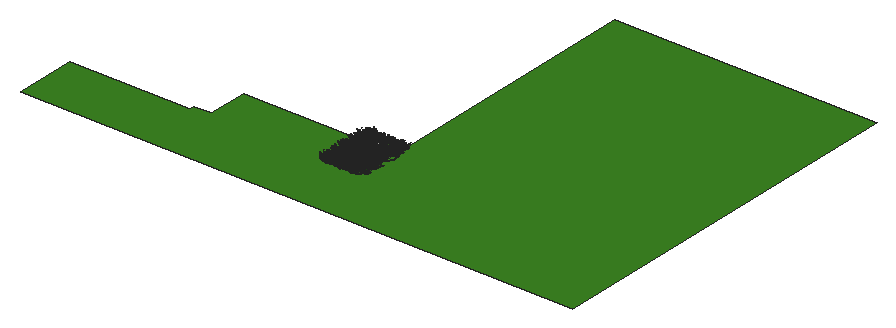
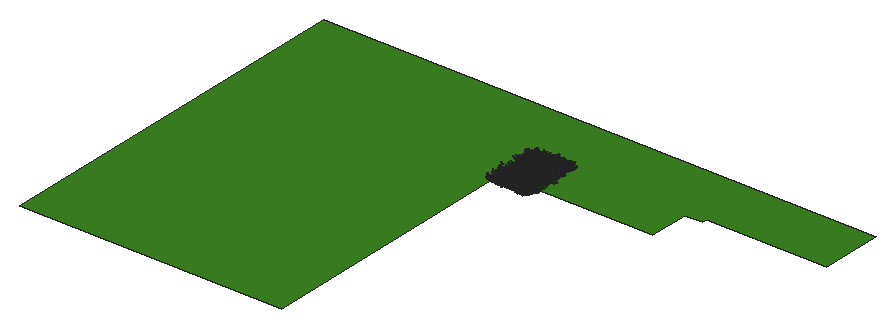
# SketchUp Ruby script. Lengths in inches.
U = 1.inch
M = Sketchup.active_model
def pt(a) = Geom::Point3d.new(a.map { |v| v * U })
def face(e, loops, mat)
  f = e.add_face(loops[0].map { |a| pt(a) })
  loops[1..].each { |l| e.add_face(l.map { |a| pt(a) }).erase! }
  f.material = f.back_material = mat if mat
  f
end
# faces: each face lists its corners as indices into pts; further lists are holes
def faces(e, pts, list, mat = nil) = list.each { |f| face(e, (f[0].is_a?(Array) ? f : [f]).map { |l| l.map { |i| pts[i] } }, mat) }
# xy, xz, yz: faces in a plane at the given z, y or x. An outline is a flat list of corners, or four numbers for a rectangle; further outlines are holes
def ring(l) = l.size == 4 ? [[l[0], l[1]], [l[2], l[1]], [l[2], l[3]], [l[0], l[3]]] : l.each_slice(2).to_a
def flat(e, list, mat, &to3) = list.each { |f| face(e, (f[0].is_a?(Array) ? f : [f]).map { |l| ring(l).map { |u, v| to3.(u, v) } }, mat) }
def xy(e, z, list, mat = nil) = flat(e, list, mat) { |x, y| [x, y, z] }
def xz(e, y, list, mat = nil) = flat(e, list, mat) { |x, z| [x, y, z] }
def yz(e, x, list, mat = nil) = flat(e, list, mat) { |y, z| [x, y, z] }
def lines(e, pts, list) = list.each { |a, b| e.add_line(pt(pts[a]), pt(pts[b])) }
# prism: a flat outline (further loops are holes) pulled along v
def prism(e, loops, v, mat = nil)
  f = face(e, loops, mat); d = Geom::Vector3d.new(v.map { |x| x * U })
  f.pushpull(f.normal.samedirection?(d) ? d.length : -d.length)
end
def box(e, o, s, mat = nil) = prism(e, [[o, [o[0] + s[0], o[1], o[2]], [o[0] + s[0], o[1] + s[1], o[2]], [o[0], o[1] + s[1], o[2]]]], [0, 0, s[2]], mat)
def at(x, y, z, deg = 0) = Geom::Transformation.translation(pt([x, y, z])) * Geom::Transformation.rotation(ORIGIN, Z_AXIS, deg.degrees)
def axes(o, x, y, z) = Geom::Transformation.new([*x, 0, *y, 0, *z, 0, *pt(o).to_a, 1])
def part(name) = M.definitions.add(name)
# library, detail: a bought-in or finely detailed component or shape, given as its bounding box
def library(name, o, s) = part(name).tap { |d| box(d.entities, o, s) }
def detail(e, o, s) = box(e.add_group.entities, o, s)
def put(e, d, t, mat = nil) = e.add_instance(d, t).tap { |i| i.material = mat if mat }
def group(e, t, mat = nil) = e.add_group.tap { |g| g.transformation = t; g.material = mat if mat }.entities
root = M.entities
M.materials.add("Material82").color = [68, 110, 58]
M.materials.add("Material83").color = [48, 90, 38]
M.materials.add("Material84").color = [68, 110, 48]
M.materials.add("Material85").color = [48, 90, 48]
M.materials.add("Material86").color = [58, 110, 58]
M.materials.add("Material87").color = [58, 90, 38]
M.materials.add("Material88").color = [68, 100, 58]
M.materials.add("Material89").color = [48, 100, 38]
M.materials.add("[Color M01]").color = [60, 133, 34]
c1 = part("grass00")
p = [[-0.6875,0.15,0],[-0.56,0.08,5.52],[-0.04,0.03,2.76],[0.48,-0.02,0],[0.35,-0.02,5.52],[-0.1,-0.14,5.52],
  [-0.12,0.65,8.37],[-0.42,0.65,8.37]]
faces(c1.entities,p,[[0,1,2,3],[3,2,4],[1,5,2],[5,4,2],[1,6,5],[4,5,6],[7,6,1]])
c2 = part("Group16\#1")
put(c2.entities,c1,axes([1.44,-0.61,-0.01],[0.05352,0.12609,0],[-0.10704,0.04543,0.07239],[0.06664,-0.02828,0.11628]),"Material85")
put(c2.entities,c1,axes([0.76,-0.15,-0.01],[0.04676,0.24062,0],[-0.23162,0.04501,0.06642],[0.0652,-0.01267,0.23595]),"Material82")
put(c2.entities,c1,axes([0.79,0.01,-0.01],[-0.00606,0.34651,0],[-0.34381,-0.00602,0.0432],[0.04319,0.00076,0.34386]))
put(c2.entities,c1,axes([1,0.23,-0.01],[-0.07192,0.31144,0],[-0.28722,-0.06632,0.1236],[0.12043,0.02781,0.29478]),"Material84")
put(c2.entities,c1,axes([1.66,0.77,-0.01],[-0.13828,0.29651,0],[-0.21551,-0.1005,0.22471],[0.20365,0.09498,0.23779]),"Material89")
put(c2.entities,c1,axes([0.6875,0.52,-0.01],[-0.18126,0.24051,0],[-0.22746,-0.17142,0.09788],[0.07817,0.05891,0.28481]),"Material84")
put(c2.entities,c1,axes([0.68,0.78,-0.01],[-0.215,0.18688,0],[-0.12385,-0.14248,0.21334],[0.13995,0.16101,0.18878]),"Material82")
put(c2.entities,c1,axes([0.56,1,-0.01],[-0.13756,0.07624,0],[-0.06159,-0.11112,0.0927],[0.04494,0.08108,0.12705]),"Material84")
put(c2.entities,c1,axes([0.2,0.64,-0.01],[-0.23729,0.07254,0],[-0.05711,-0.18681,0.153],[0.04473,0.14632,0.19535]),"Material89")
put(c2.entities,c1,axes([0.0625,0.72,-0.01],[-0.28874,0.02525,0],[-0.02179,-0.24916,0.14647],[0.01276,0.14591,0.25012]),"Material82")
put(c2.entities,c1,axes([-0.08,0.62,-0.01],[-0.34089,-0.04187,0],[0.03255,-0.26504,0.216],[-0.02633,0.21439,0.26703]),"Material89")
put(c2.entities,c1,axes([-0.34,0.98,-0.01],[-0.14314,-0.0493,0],[0.04397,-0.12769,0.06843],[-0.02228,0.0647,0.13505]),"Material89")
put(c2.entities,c1,axes([-0.87,1.45,-0.01],[-0.23488,-0.14114,0],[0.13761,-0.22901,0.06087],[-0.03135,0.05217,0.26717]))
put(c2.entities,c1,axes([-0.72,0.77,-0.01],[-0.14208,-0.13251,0],[0.07209,-0.0773,0.16301],[-0.11118,0.11922,0.1057]),"Material89")
put(c2.entities,c1,axes([-0.62,0.43,-0.01],[-0.14845,-0.21203,0],[0.18654,-0.13061,0.12304],[-0.10079,0.07057,0.22772]),"Material82")
put(c2.entities,c1,axes([-0.68,0.29,-0.01],[-0.13639,-0.32136,0],[0.31723,-0.13464,0.05579],[-0.05136,0.0218,0.34462]),"Material83")
put(c2.entities,c1,axes([-0.64,0.125,-0.01],[-0.0458,-0.23569,0],[0.22124,-0.043,0.08276],[-0.08124,0.01579,0.22538]),"Material86")
put(c2.entities,c1,axes([-1.6,-0.03,-0.01],[0.00576,-0.32897,0],[0.27526,0.00482,0.18018],[-0.18015,-0.00315,0.2753]),"Material84")
put(c2.entities,c1,axes([-1.36,-0.31,-0.01],[0.05718,-0.24765,0],[0.18172,0.04196,0.17267],[-0.16825,-0.03885,0.1865]),"Material89")
put(c2.entities,c1,axes([-1.54,-0.72,-0.01],[0.06537,-0.14017,0],[0.13555,0.06321,0.03939],[-0.0357,-0.01665,0.14956]))
put(c2.entities,c1,axes([-1.19,-0.9,-0.01],[0.09597,-0.12735,0],[0.11214,0.08451,0.07557],[-0.06035,-0.04548,0.14042]),"Material88")
put(c2.entities,c1,axes([-0.47,-0.54,-0.01],[0.11588,-0.10072,0],[0.0618,0.0711,0.12124],[-0.07953,-0.0915,0.0942]))
put(c2.entities,c1,axes([-0.47,-0.84,-0.01],[0.11927,-0.0661,0],[0.06603,0.11913,0.00646],[-0.00313,-0.00565,0.13621]),"Material84")
put(c2.entities,c1,axes([-0.38,-1.24,-0.01],[0.28037,-0.08571,0],[0.0618,0.20215,0.20315],[-0.05939,-0.19428,0.21139]),"Material88")
put(c2.entities,c1,axes([-0.06,-0.66,-0.01],[0.22719,-0.01987,0],[0.01247,0.14255,0.17758],[-0.01547,-0.17691,0.1431]),"Material87")
put(c2.entities,c1,axes([0.11,-0.89,-0.01],[0.14882,0.01828,0],[-0.01058,0.08611,0.12229],[0.01491,-0.12138,0.08676]),"Material85")
put(c2.entities,c1,axes([0.25,-0.72,-0.01],[0.20481,0.07053,0],[-0.06206,0.18022,0.10291],[0.03351,-0.0973,0.1906]),"Material85")
put(c2.entities,c1,axes([0.85,-1.42,-0.01],[0.16481,0.09904,0],[-0.09472,0.15762,0.05616],[0.02893,-0.04814,0.18389]),"Material84")
put(c2.entities,c1,axes([1.01,-1.09,-0.01],[0.21858,0.20385,0],[-0.17495,0.1876,0.15339],[0.10462,-0.11218,0.25652]),"Material89")
put(c2.entities,c1,axes([1.01,-0.71,-0.01],[0.08733,0.12473,0],[-0.06445,0.04512,0.13037],[0.1068,-0.07477,0.07867]),"Material85")
c3 = part("Group15\#1")
put(c3.entities,c2,at(0,0,0))
c4 = part("3darcstudiotree_grass00\#1")
put(c4.entities,c3,at(0,0,0))
xy(root,-29.74,[[486.07,932.5,1048.3125,932.5,1048.3125,1318.18,782.4375,1318.18,782.4375,1040.81,626.34,1040.81,626.34,1000.12,608.75,1000.12,608.75,994.94,486.07,994.94]],"[Color M01]")
put(root,c4,axes([747.01,1042.55,-29.74],[0.6827,1.82438,0],[-3.27697,0.19072,-0.00575],[-0.03023,0.00176,1.31904]))
put(root,c4,axes([747.21,997.3,-29.74],[0.45996,1.33665,0],[-3.57607,0.19139,-0.02967],[-0.17102,0.00915,1.57371]))
put(root,c4,axes([749.13,1041.28,-29.74],[-3.10229,-1.16988,0],[2.93363,-1.20992,-0.00934],[0.03186,-0.01314,1.57129]))
put(root,c4,axes([747.14,1024.93,-29.74],[2.66376,1.48543,0],[-3.56736,0.99495,-0.03132],[-0.13982,0.039,1.7905]))
put(root,c4,axes([749.33,1044.75,-29.74],[-2.84959,-0.68183,0],[2.166,-1.40791,-0.04577],[0.14869,-0.09665,1.96036]))
put(root,c4,axes([749.8125,1042.05,-29.74],[-4.12072,-0.27119,0],[0.6549,-1.54771,-0.03361],[0.02858,-0.06755,1.54092]))
put(root,c4,axes([749.8,996.66,-29.74],[-2.73846,-0.74739,0],[2.06192,-1.17502,-0.03348],[0.13147,-0.07492,1.87437]))
put(root,c4,axes([750.14,1027.05,-29.74],[-1.65449,-1.67632,0],[3.5536,-0.54549,-0.00938],[0.04968,-0.00763,1.62403]))
put(root,c4,axes([750.26,1016.8125,-29.74],[-2.10435,-1.3155,0],[3.64518,-0.9069,-0.04882],[0.17684,-0.044,1.38366]))
put(root,c4,axes([750.13,1033.6,-29.74],[-3.62624,-0.35306,0],[1.02554,-1.63824,-0.03453],[0.0374,-0.05975,1.44935]))
put(root,c4,axes([749.03,1039.09,-29.74],[0.82539,1.5958,0],[-3.41483,0.2747,-0.03877],[-0.28197,0.02268,1.93915]))
put(root,c4,axes([749.41,1011.43,-29.74],[3.93831,-0.79818,0],[2.14355,1.64496,-0.04443],[0.08068,0.06192,1.39643]))
put(root,c4,axes([750.67,1020.12,-29.74],[-2.03778,-1.0951,0],[3.7049,-1.07224,-0.05528],[0.23064,-0.06675,1.78248]))
put(root,c4,axes([750.68,1019.15,-29.74],[-3.67688,-0.6634,0],[1.45076,-1.25058,-0.02741],[0.08145,-0.07021,1.86713]))
put(root,c4,axes([749.05,1023.27,-29.74],[3.8654,0.35733,0],[-0.81256,1.36706,-0.007],[-0.00937,0.01576,1.56436]))
put(root,c4,axes([749.31,1029.81,-29.74],[0.38941,1.44392,0],[-4.06327,0.17043,-0.05804],[-0.26328,0.01104,1.39706]))
put(root,c4,axes([749.3,1050.98,-29.74],[3.44355,0.26807,0],[-0.70938,1.41724,-0.02055],[-0.0272,0.05435,1.87683]))
put(root,c4,axes([751.07,1007.75,-29.74],[-3.021,-0.6477,0],[1.60996,-1.16789,-0.02167],[0.0547,-0.03968,1.33527]))
put(root,c4,axes([750.93,1036.58,-29.74],[-4.07234,0.0884,0],[-0.21728,-1.55677,-0.00024],[-0.00008,-0.0006,1.85086]))
put(root,c4,axes([750.67,999.31,-29.74],[-3.52536,0.66718,0],[-1.57507,-1.29441,-0.02803],[-0.08559,-0.07034,1.92571]))
put(root,c4,axes([749.79,1053.3125,-29.74],[0.25287,1.52902,0],[-3.62555,0.09325,-0.03468],[-0.21891,0.00563,1.72254]))
put(root,c4,axes([750.23,1014.4375,-29.74],[3.86172,-0.56351,0],[1.21864,1.29888,-0.04569],[0.10723,0.11428,1.78027]))
put(root,c4,axes([751.52,1049.22,-29.74],[-4.49885,0.1512,0],[-0.3136,-1.45126,-0.04489],[-0.02566,-0.11876,1.86365]))
put(root,c4,axes([751.02,1009.58,-29.74],[2.47969,-0.8558,0],[2.79846,1.26111,-0.0129],[0.03707,0.01671,1.39029]))
put(root,c4,axes([750.74,1025.95,-29.74],[3.77184,-0.74152,0],[2.04611,1.61872,-0.00236],[0.0043,0.00341,1.40454]))
put(root,c4,axes([751.9375,1047.68,-29.74],[-3.95195,-0.11479,0],[0.31612,-1.69258,-0.00991],[0.00383,-0.02049,1.69565]))
put(root,c4,axes([750.69,1003.09,-29.74],[4.4523,-0.10128,0],[0.21715,1.4846,-0.03809],[0.01394,0.09529,1.79573]))
put(root,c4,axes([751.125,1001.68,-29.74],[3.96943,-0.89247,0],[1.86138,1.2876,-0.05304],[0.17378,0.12021,1.86337]))
put(root,c4,axes([752.54,1005.29,-29.74],[-0.06079,-1.40056,0],[3.30003,-0.02228,-0.01279],[0.0855,-0.00058,1.65408]))
put(root,c4,axes([752.48,1031.88,-29.74],[-0.47592,1.56401,0],[-3.26389,-0.15447,-0.01529],[-0.10295,-0.00487,1.67142]))
put(root,c4,axes([754.48,1006.18,-29.74],[-0.30634,-1.35211,0],[4.22133,-0.14875,-0.01785],[0.10663,-0.00376,1.90542]))
put(root,c4,axes([754.57,1006.96,-29.74],[0.00917,-1.7323,0],[3.83355,0.00316,-0.00952],[0.04811,0.00004,1.45276]))
put(root,c4,axes([755.09,1031.06,-29.74],[-3.94041,-0.17555,0],[0.52244,-1.82386,-0.03054],[0.01805,-0.06303,1.83699]))
put(root,c4,axes([755.2,1038.49,-29.74],[-3.62534,0.37466,0],[-0.93047,-1.40031,-0.00505],[-0.0081,-0.01218,1.74136]))
put(root,c4,axes([754.51,1022.87,-29.74],[3.51422,-0.54071,0],[1.19989,1.21289,-0.03886],[0.08676,0.0877,1.52001]))
put(root,c4,axes([756.16,1051.37,-29.74],[-3.51186,-0.721,0],[1.80955,-1.37083,-0.02288],[0.05511,-0.04175,1.53217]))
put(root,c4,axes([756.18,1029.875,-29.74],[1.44921,-1.37247,0],[3.47001,0.56986,-0.04485],[0.23379,0.03839,1.59096]))
put(root,c4,axes([755.31,1002.98,-29.74],[0.66388,1.42145,0],[-3.998,0.29041,-0.0472],[-0.22325,0.01622,1.46547]))
put(root,c4,axes([755.41,1025.51,-29.74],[2.60904,1.49403,0],[-2.88542,0.78369,-0.04649],[-0.18984,0.05156,1.30192]))
put(root,c4,axes([755.52,1013.72,-29.74],[3.83063,0.28141,0],[-0.63066,1.33518,-0.03922],[-0.04064,0.08605,1.46066]))
put(root,c4,axes([756.07,1028.07,-29.74],[2.98326,-0.56932,0],[1.56375,1.27443,-0.0104],[0.02417,0.0197,1.43546]))
put(root,c4,axes([755.47,1039.72,-29.74],[0.44153,1.60869,0],[-4.59886,0.19631,-0.03135],[-0.13775,0.00588,1.53244]))
put(root,c4,axes([756.1,1042.45,-29.74],[3.7963,-0.32727,0],[0.82791,1.49367,-0.02018],[0.02229,0.04022,1.50307]))
put(root,c4,axes([758.06,1018.1,-29.74],[-2.44222,-1.21448,0],[3.27109,-1.02306,-0.01126],[0.03735,-0.01168,1.32461]))
put(root,c4,axes([757.73,1012.8,-29.74],[-3.39135,-0.3159,0],[0.83318,-1.39116,-0.01801],[0.02035,-0.03397,1.33554]))
put(root,c4,axes([757.61,1009.53,-29.74],[-1.25644,-1.35671,0],[3.16457,-0.45581,-0.03784],[0.23357,-0.03364,1.65933]))
put(root,c4,axes([758,1046.6,-29.74],[-0.2827,-1.72948,0],[4.63241,-0.11777,-0.03565],[0.15653,-0.00398,1.53082]))
put(root,c4,axes([758.16,1020.64,-29.74],[-4.6912,-0.24024,0],[0.57575,-1.74859,-0.02421],[0.01544,-0.0469,1.66024]))
put(root,c4,axes([757.25,1045.24,-29.74],[2.39093,-1.03283,0],[3.02488,1.08907,-0.05494],[0.24262,0.08735,1.83588]))
put(root,c4,axes([757.28,1001.06,-29.74],[3.97766,0.18345,0],[-0.40911,1.37962,-0.0104],[-0.00856,0.02886,1.87036]))
put(root,c4,axes([758.13,1036.82,-29.74],[2.63553,-1.14097,0],[3.49929,1.25715,-0.04921],[0.17097,0.06142,1.66765]))
put(root,c4,axes([758,1034.22,-29.74],[-2.26024,1.36544,0],[-3.77789,-0.97262,-0.02867],[-0.12669,-0.03262,1.78429]))
put(root,c4,axes([757.52,997.26,-29.74],[2.88281,0.64392,0],[-1.76321,1.22772,-0.02459],[-0.08623,0.06004,1.90817]))
put(root,c4,axes([758.22,1016.9375,-29.74],[3.80429,-0.95187,0],[2.21902,1.37934,-0.04672],[0.14892,0.09257,1.84728]))
put(root,c4,axes([757.61,998.35,-29.74],[3.38308,1.28097,0],[-3.13031,1.28579,-0.04664],[-0.1697,0.06971,1.77978]))
put(root,c4,axes([758.21,1048.77,-29.74],[1.17272,1.70605,0],[-3.75992,0.40197,-0.02312],[-0.1149,0.01228,1.50331]))
put(root,c4,axes([760.57,1020.29,-29.74],[2.08515,-1.11593,0],[3.14779,0.91479,-0.04551],[0.20545,0.05971,1.64335]))
put(root,c4,axes([760.6,1014.2,-29.74],[-2.84594,1.17329,0],[-3.06349,-1.15571,-0.01205],[-0.05136,-0.01938,1.87482]))
put(root,c4,axes([761.64,1004.18,-29.74],[-4.1718,-0.04402,0],[0.1133,-1.66995,-0.01377],[0.00192,-0.02825,1.65227]))
put(root,c4,axes([761.21,1028.09,-29.74],[-3.19418,0.83767,0],[-2.09756,-1.24397,-0.00165],[-0.00457,-0.00271,1.42237]))
put(root,c4,axes([762.15,1009.56,-29.74],[-3.23677,-0.61439,0],[2.0349,-1.66734,-0.00367],[0.00726,-0.00595,1.60507]))
put(root,c4,axes([761.77,1001.03,-29.74],[0.66157,-1.84804,0],[3.88634,0.21638,-0.01886],[0.11067,0.00616,1.74385]))
put(root,c4,axes([760.78,1024.71,-29.74],[3.70848,0.20038,0],[-0.48617,1.3994,-0.00884],[-0.00845,0.02433,1.89082]))
put(root,c4,axes([760.92,1049.92,-29.74],[3.47876,0.69717,0],[-2.07434,1.60981,-0.02666],[-0.05222,0.04053,1.48409]))
put(root,c4,axes([761.49,998.35,-29.74],[-1.68767,1.14523,0],[-4.10192,-0.94014,-0.02835],[-0.11929,-0.02734,1.73088]))
put(root,c4,axes([762.9375,1042.89,-29.74],[-4.10821,-0.63147,0],[1.40621,-1.42285,-0.03755],[0.0732,-0.07407,1.55797]))
put(root,c4,axes([761.49,1039.9,-29.74],[4.36048,0.20882,0],[-0.42656,1.38529,-0.01966],[-0.01597,0.05186,1.78732]))
put(root,c4,axes([761.93,1031.31,-29.74],[-1.75851,1.2095,0],[-3.69968,-0.83659,-0.01882],[-0.09945,-0.02249,1.94745]))
put(root,c4,axes([763.47,1038.96,-29.74],[-1.44336,-1.26835,0],[3.91991,-0.69378,-0.01184],[0.05292,-0.00937,1.57815]))
put(root,c4,axes([763.24,1044.71,-29.74],[-0.45128,-1.33361,0],[4.22591,-0.22241,-0.03174],[0.17504,-0.00921,1.77768]))
put(root,c4,axes([762.29,1007.53,-29.74],[3.82795,-0.89848,0],[2.12017,1.40489,-0.02674],[0.0662,0.04387,1.50406]))
put(root,c4,axes([763.36,1047.18,-29.74],[-2.48368,-1.57939,0],[3.38438,-0.82775,-0.05324],[0.27998,-0.06848,1.84703]))
put(root,c4,axes([763.24,1022.47,-29.74],[-3.70161,0.1835,0],[-0.55617,-1.74492,-0.04842],[-0.0352,-0.11043,1.94818]))
put(root,c4,axes([763.78,996.95,-29.74],[-2.02199,-1.57321,0],[3.0284,-0.60536,-0.03791],[0.25064,-0.0501,1.88609]))
put(root,c4,axes([762.4375,1019.16,-29.74],[4.60425,0.18746,0],[-0.4763,1.81947,-0.06196],[-0.02818,0.10763,1.53928]))
put(root,c4,axes([762.65,1005.1,-29.74],[3.66376,0.25232,0],[-0.75626,1.7079,-0.04039],[-0.02947,0.06656,1.39779]))
put(root,c4,axes([762.9,1016.97,-29.74],[3.38223,0.96892,0],[-2.45655,1.33368,-0.05492],[-0.16887,0.09168,1.63919]))
put(root,c4,axes([764.09,1050.81,-29.74],[-3.51929,1.02852,0],[-2.47816,-1.3188,-0.03727],[-0.13373,-0.07117,1.88005]))
put(root,c4,axes([763.54,1030.35,-29.74],[3.59827,-1.20315,0],[2.55541,1.18863,-0.04452],[0.1901,0.08842,1.95574]))
put(root,c4,axes([762.75,1034.56,-29.74],[2.55345,1.05656,0],[-3.3838,1.27189,-0.0237],[-0.06613,0.02486,1.35093]))
put(root,c4,axes([763.8,1012.71,-29.74],[3.17823,1.19717,0],[-2.46254,1.01678,-0.00574],[-0.02103,0.00868,1.41814]))
put(root,c4,axes([764,1036.57,-29.74],[1.4209,1.26091,0],[-3.92098,0.6872,-0.00487],[-0.02309,0.00405,1.66894]))
put(root,c4,axes([766.67,1001.15,-29.74],[-4.20115,-0.27572,0],[0.6063,-1.43684,-0.03971],[0.03476,-0.08238,1.4765]))
put(root,c4,axes([766.01,1047.37,-29.74],[-2.56197,0.85481,0],[-2.91428,-1.35846,-0.04396],[-0.15305,-0.07134,1.82298]))
put(root,c4,axes([766.08,1048.45,-29.74],[-3.07207,1.32257,0],[-2.98229,-1.07739,-0.02313],[-0.10886,-0.03933,1.93523]))
put(root,c4,axes([766.07,1007.88,-29.74],[3.03154,-1.30842,0],[2.70015,0.973,-0.04297],[0.17128,0.06172,1.48019]))
put(root,c4,axes([765.98,1010.51,-29.74],[4.0708,-0.43574,0],[1.12817,1.63922,-0.0215],[0.0298,0.0433,1.70776]))
put(root,c4,axes([765.75,1035.875,-29.74],[1.45585,1.40356,0],[-4.29762,0.69331,-0.06498],[-0.33385,0.05386,1.93183]))
put(root,c4,axes([766.31,1021.4,-29.74],[3.98961,-0.74286,0],[1.49364,1.24762,-0.01833],[0.03992,0.03334,1.33779]))
put(root,c4,axes([766.23,1023.45,-29.74],[-1.90909,1.29111,0],[-3.77719,-0.86865,-0.00159],[-0.00678,-0.00156,1.61385]))
put(root,c4,axes([766.16,1042.29,-29.74],[3.44974,0.13102,0],[-0.35474,1.45265,-0.03978],[-0.02715,0.11118,1.9745]))
put(root,c4,axes([766.79,1031.26,-29.74],[4.01141,-0.57098,0],[1.38004,1.50792,-0.00463],[0.00922,0.01007,1.7876]))
put(root,c4,axes([768.29,999.71,-29.74],[-2.56515,-0.8375,0],[2.7288,-1.2999,-0.02106],[0.06081,-0.02897,1.45262]))
put(root,c4,axes([766.27,1017.93,-29.74],[1.21271,1.28553,0],[-4.16441,0.61099,-0.01219],[-0.04469,0.00656,1.30286]))
put(root,c4,axes([767.52,1011.61,-29.74],[-3.04036,1.06501,0],[-2.34315,-1.04035,-0.02123],[-0.07304,-0.03243,1.37003]))
put(root,c4,axes([767.73,1017.28,-29.74],[1.27723,-1.67859,0],[3.60633,0.42678,-0.0465],[0.22987,0.0272,1.45674]))
put(root,c4,axes([766.8,1005.15,-29.74],[4.09443,-0.06366,0],[0.15428,1.54325,-0.03451],[0.00867,0.0867,1.8714]))
put(root,c4,axes([768.57,1051.75,-29.74],[-2.71598,-1.39793,0],[3.51357,-1.0617,-0.04805],[0.18587,-0.05616,1.61679]))
put(root,c4,axes([766.75,1003.16,-29.74],[3.43879,0.48398,0],[-1.47194,1.62658,-0.03925],[-0.05225,0.05774,1.29995]))
put(root,c4,axes([768.13,1044.11,-29.74],[0.94515,-1.66762,0],[4.07339,0.35906,-0.0396],[0.18346,0.01617,1.48525]))
put(root,c4,axes([767.67,1034.39,-29.74],[2.86215,-0.69885,0],[2.15737,1.37418,-0.03178],[0.09016,0.05743,1.65559]))
put(root,c4,axes([767.39,1039.95,-29.74],[2.07536,1.00802,0],[-2.97078,0.95128,-0.04172],[-0.20153,0.06453,1.78477]))
put(root,c4,axes([768.93,1037.93,-29.74],[0.03648,-1.32003,0],[3.51668,0.01511,-0.01263],[0.08154,0.00035,1.70174]))
put(root,c4,axes([769.15,1013.93,-29.74],[-0.06785,-1.57512,0],[4.70678,-0.03153,-0.0635],[0.34719,-0.00233,1.92948]))
put(root,c4,axes([768.79,1027.73,-29.74],[-0.80195,1.7338,0],[-4.65742,-0.33505,-0.02378],[-0.12913,-0.00929,1.95907]))
put(root,c4,axes([769.1,997.23,-29.74],[-1.48177,1.26839,0],[-3.97677,-0.72256,-0.00587],[-0.02393,-0.00435,1.47291]))
put(root,c4,axes([769.13,1028.88,-29.74],[4.46941,0.03034,0],[-0.07094,1.62545,-0.04862],[-0.00377,0.08633,1.39123]))
put(root,c4,axes([769.6,1024.98,-29.74],[3.5964,-0.66598,0],[1.43149,1.20228,-0.03796],[0.09777,0.08212,1.52986]))
put(root,c4,axes([771.54,1007.8,-29.74],[-3.83088,0.01586,0],[-0.04003,-1.50367,-0.01485],[-0.00089,-0.03334,1.62647]))
put(root,c4,axes([771.44,1036.53,-29.74],[2.50638,-0.90958,0],[2.96207,1.26944,-0.00074],[0.00258,0.00111,1.68668]))
put(root,c4,axes([772.05,1021.55,-29.74],[-1.26463,-1.25515,0],[3.81596,-0.59798,-0.04918],[0.19961,-0.03128,1.34418]))
put(root,c4,axes([771.48,1029.59,-29.74],[-2.59269,1.36416,0],[-3.43206,-1.0145,-0.01976],[-0.08545,-0.02526,1.7373]))
put(root,c4,axes([771.25,1031.63,-29.74],[4.23995,-0.14734,0],[0.39715,1.77755,-0.00682],[0.00263,0.01179,1.49182]))
put(root,c4,axes([772.49,1023.46,-29.74],[0.54946,-1.30633,0],[4.42126,0.28923,-0.06063],[0.27406,0.01793,1.53907]))
put(root,c4,axes([771.35,1045.02,-29.74],[4.19345,0.64908,0],[-1.43857,1.4455,-0.00074],[-0.00143,0.00144,1.56313]))
put(root,c4,axes([773.32,1033.59,-29.74],[-4.00947,-0.30727,0],[0.87061,-1.76683,-0.00093],[0.00074,-0.0015,1.42207]))
put(root,c4,axes([773.45,1042.25,-29.74],[-2.04014,-1.04561,0],[3.14641,-0.95481,-0.03027],[0.11908,-0.03613,1.47708]))
put(root,c4,axes([771.7,1027.68,-29.74],[0.66214,1.69294,0],[-3.60919,0.21955,-0.0058],[-0.03794,0.00231,1.813]))
put(root,c4,axes([772.95,996.64,-29.74],[-3.15684,0.83052,0],[-1.94414,-1.14932,-0.03251],[-0.12313,-0.07279,1.79208]))
put(root,c4,axes([773.18,1011.55,-29.74],[1.45773,-1.41559,0],[3.72691,0.5969,-0.04502],[0.25742,0.04123,1.86083]))
put(root,c4,axes([772.86,1001.95,-29.74],[3.14963,-1.20842,0],[2.29792,0.93151,-0.01443],[0.07601,0.03081,1.86565]))
put(root,c4,axes([774.02,1015.89,-29.74],[-4.00454,-0.52801,0],[1.05814,-1.24816,-0.00172],[0.00311,-0.00367,1.42531]))
put(root,c4,axes([774.12,1002.76,-29.74],[-1.0046,-1.54951,0],[3.94346,-0.39764,-0.04783],[0.24428,-0.02463,1.6084]))
put(root,c4,axes([774.44,1040.2,-29.74],[-2.23262,-1.3088,0],[3.58665,-0.95157,-0.0439],[0.1738,-0.04611,1.54604]))
put(root,c4,axes([772.62,1025.83,-29.74],[2.75664,0.78459,0],[-2.60411,1.42301,-0.01696],[-0.0547,0.02989,1.8379]))
put(root,c4,axes([772.84,1015.01,-29.74],[1.57656,1.15501,0],[-3.7913,0.80487,-0.00648],[-0.02974,0.00631,1.68262]))
put(root,c4,axes([774.65,1051.72,-29.74],[-4.26955,0.05297,0],[-0.11438,-1.43394,-0.03177],[-0.00727,-0.09116,1.98473]))
put(root,c4,axes([773.04,1046.57,-29.74],[3.41924,1.14131,0],[-2.67356,1.24575,-0.04954],[-0.1842,0.08583,1.78537]))
put(root,c4,axes([775.13,1004.75,-29.74],[-0.37683,-1.42813,0],[4.6236,-0.18974,-0.00351],[0.01488,-0.00061,1.48465]))
put(root,c4,axes([773.34,999.82,-29.74],[4.54007,0.12562,0],[-0.30482,1.71344,-0.05051],[-0.02069,0.11631,1.91076]))
put(root,c4,axes([775.14,1049.48,-29.74],[-2.30012,-1.16982,0],[2.63485,-0.80575,-0.0081],[0.04804,-0.01469,1.87526]))
put(root,c4,axes([774.78,1038.24,-29.74],[0.45602,-1.75469,0],[4.51141,0.18235,-0.06373],[0.28019,0.01133,1.50237]))
put(root,c4,axes([774.74,1009.14,-29.74],[1.62707,-1.18617,0],[3.8873,0.82932,-0.03985],[0.15889,0.0339,1.5017]))
put(root,c4,axes([774.3,1018.41,-29.74],[4.17569,0.70475,0],[-1.86329,1.71705,-0.06274],[-0.13365,0.12316,1.92197]))
put(root,c4,axes([776.7,1010.7,-29.74],[-3.80347,-0.79702,0],[1.88494,-1.39901,-0.03648],[0.10192,-0.07565,1.79293]))
put(root,c4,axes([776.64,1008.4,-29.74],[-2.17021,-1.46243,0],[2.84473,-0.65657,-0.0221],[0.14072,-0.03248,1.82262]))
put(root,c4,axes([776.68,999.1,-29.74],[3.21046,-0.42194,0],[1.31397,1.55496,-0.01535],[0.02427,0.02872,1.5577]))
put(root,c4,axes([777.97,1040.96,-29.74],[-3.29126,-0.79109,0],[1.80045,-1.16502,-0.03312],[0.11366,-0.07354,1.70984]))
put(root,c4,axes([777.65,1044.58,-29.74],[0.99321,-1.58581,0],[3.96504,0.38623,-0.04714],[0.20087,0.01957,1.34372]))
put(root,c4,axes([778.21,1012.83,-29.74],[-2.18591,-1.17845,0],[3.11783,-0.89946,-0.02018],[0.10185,-0.02938,1.81061]))
put(root,c4,axes([776.89,1026.88,-29.74],[4.09864,-0.14348,0],[0.37168,1.65134,-0.01913],[0.00999,0.04439,1.86132]))
put(root,c4,axes([778.59,1036.55,-29.74],[-2.13357,-1.0721,0],[3.45076,-1.06807,-0.04646],[0.2021,-0.06255,1.81816]))
put(root,c4,axes([776.76,1050.68,-29.74],[3.51961,1.01739,0],[-2.56437,1.37974,-0.04132],[-0.14142,0.07609,1.88254]))
put(root,c4,axes([777.5,1014.65,-29.74],[-1.78032,1.61918,0],[-3.86174,-0.66038,-0.00354],[-0.01693,-0.0029,1.64409]))
